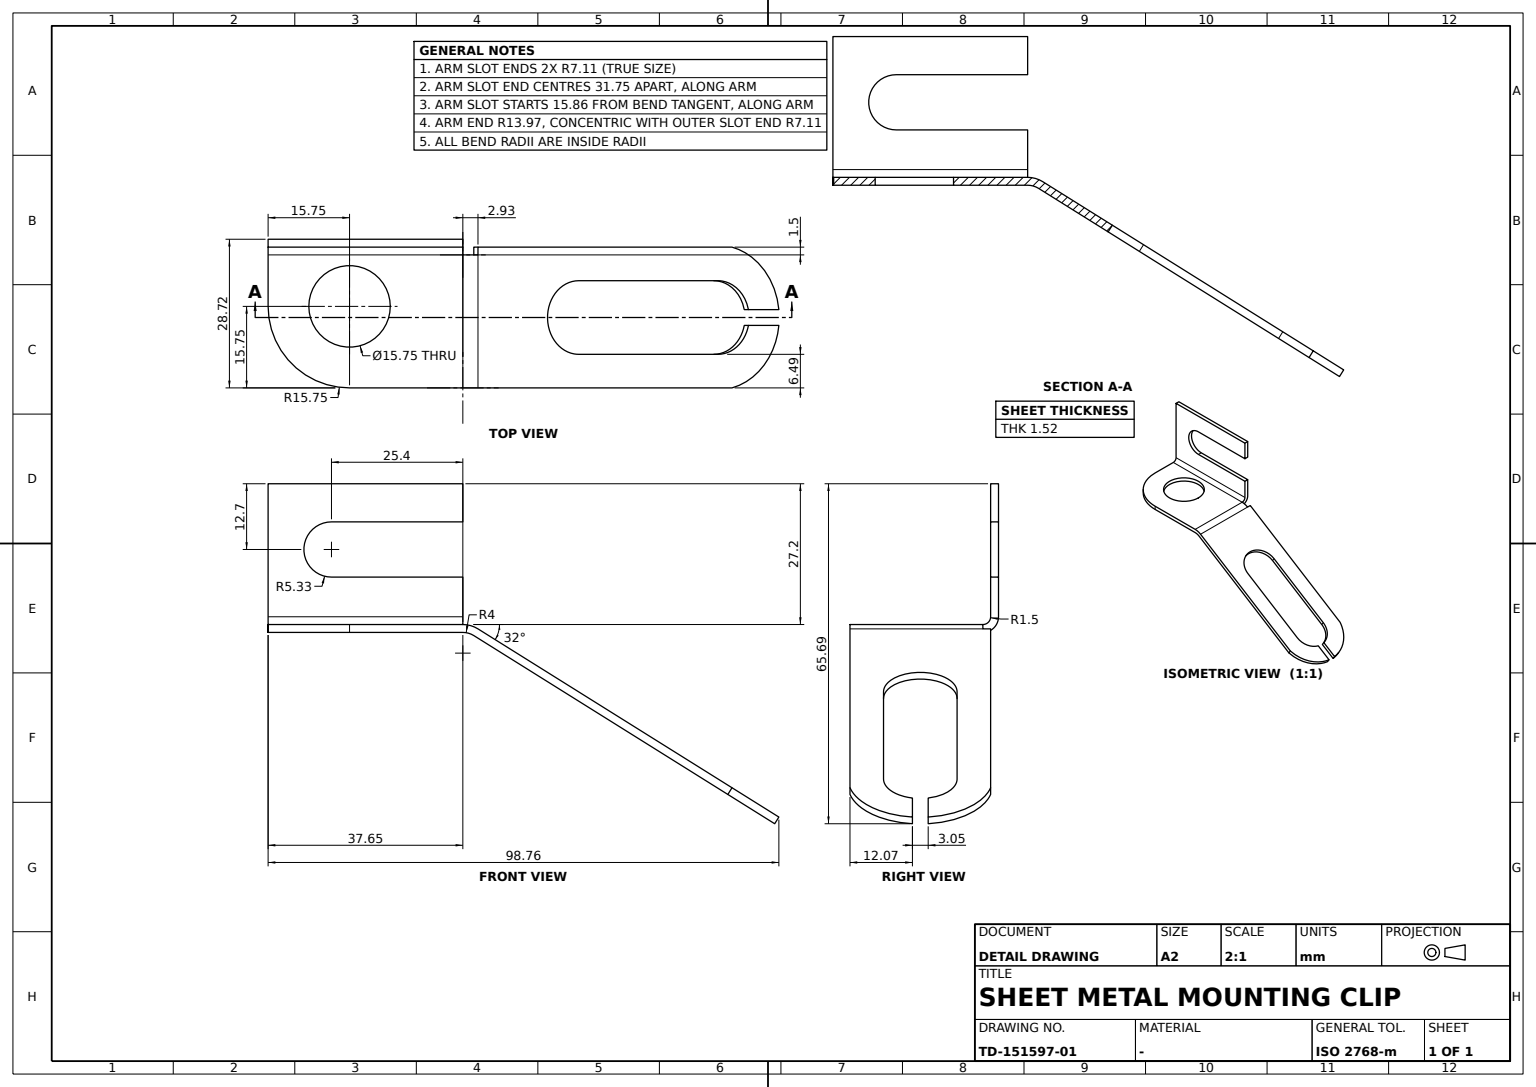
ISO-10303-21;
HEADER;
FILE_DESCRIPTION((''),'2;1');
FILE_NAME('','',(''),(''),'','','');
FILE_SCHEMA(('AUTOMOTIVE_DESIGN'));
ENDSEC;
DATA;
#1=APPLICATION_CONTEXT('');
#2=PRODUCT_CONTEXT('',#1,'mechanical');
#3=PRODUCT('','','',(#2));
#4=PRODUCT_DEFINITION_FORMATION('','',#3);
#5=PRODUCT_DEFINITION_CONTEXT('',#1,'design');
#6=PRODUCT_DEFINITION('','',#4,#5);
#7=PRODUCT_DEFINITION_SHAPE('','',#6);
#8=(LENGTH_UNIT()NAMED_UNIT(*)SI_UNIT(.MILLI.,.METRE.));
#9=(NAMED_UNIT(*)PLANE_ANGLE_UNIT()SI_UNIT($,.RADIAN.));
#10=(NAMED_UNIT(*)SI_UNIT($,.STERADIAN.)SOLID_ANGLE_UNIT());
#11=UNCERTAINTY_MEASURE_WITH_UNIT(LENGTH_MEASURE(0.005),#8,'distance_accuracy_value','');
#12=(GEOMETRIC_REPRESENTATION_CONTEXT(3)GLOBAL_UNCERTAINTY_ASSIGNED_CONTEXT((#11))GLOBAL_UNIT_ASSIGNED_CONTEXT((#8,#9,#10))REPRESENTATION_CONTEXT('',''));
#13=CARTESIAN_POINT('',(-26.546982,13.5977,21.356));
#14=VERTEX_POINT('',#13);
#15=CARTESIAN_POINT('',(-26.546982,15.1217,21.356));
#16=VERTEX_POINT('',#15);
#17=DIRECTION('',(0.,1.,0.));
#18=VECTOR('',#17,1000.);
#19=LINE('',#13,#18);
#20=EDGE_CURVE('',#14,#16,#19,.T.);
#21=ORIENTED_EDGE('',*,*,#20,.F.);
#22=CARTESIAN_POINT('',(-26.546982,13.5977,10.688));
#23=VERTEX_POINT('',#22);
#24=CARTESIAN_POINT('',(-26.546982,13.5977,16.022));
#25=DIRECTION('',(0.,0.,1.));
#26=AXIS2_PLACEMENT_3D('',#24,#17,#25);
#27=CIRCLE('',#26,5.334);
#28=EDGE_CURVE('',#23,#14,#27,.T.);
#29=ORIENTED_EDGE('',*,*,#28,.F.);
#30=CARTESIAN_POINT('',(-26.546982,15.1217,10.688));
#31=VERTEX_POINT('',#30);
#32=LINE('',#22,#18);
#33=EDGE_CURVE('',#31,#23,#32,.F.);
#34=ORIENTED_EDGE('',*,*,#33,.F.);
#35=CARTESIAN_POINT('',(-26.546982,15.1217,16.022));
#36=AXIS2_PLACEMENT_3D('',#35,#17,#25);
#37=CIRCLE('',#36,5.334);
#38=EDGE_CURVE('',#31,#16,#37,.T.);
#39=ORIENTED_EDGE('',*,*,#38,.T.);
#40=EDGE_LOOP('',(#21,#29,#34,#39));
#41=FACE_BOUND('',#40,.T.);
#42=DIRECTION('',(-1.,0.,0.));
#43=AXIS2_PLACEMENT_3D('',#24,#17,#42);
#44=CYLINDRICAL_SURFACE('',#43,5.334);
#45=ADVANCED_FACE('',(#41),#44,.F.);
#46=CARTESIAN_POINT('',(1.780292,-13.5977,0.684618));
#47=VERTEX_POINT('',#46);
#48=CARTESIAN_POINT('',(50.901496,-13.5977,-30.009717));
#49=VERTEX_POINT('',#48);
#50=CARTESIAN_POINT('',(31.407897,-13.5977,-17.828764));
#51=DIRECTION('',(0.848048096,0.,-0.529919264));
#52=VECTOR('',#51,1000.);
#53=LINE('',#50,#52);
#54=EDGE_CURVE('',#47,#49,#53,.T.);
#55=ORIENTED_EDGE('',*,*,#54,.T.);
#56=CARTESIAN_POINT('',(59.961161,-1.524,-35.670824));
#57=VERTEX_POINT('',#56);
#58=CARTESIAN_POINT('',(48.184636,0.,-28.312035));
#59=DIRECTION('',(0.529919264,0.,0.848048096));
#60=AXIS2_PLACEMENT_3D('',#58,#59,#51);
#61=CIRCLE('',#60,13.97);
#62=EDGE_CURVE('',#49,#57,#61,.T.);
#63=ORIENTED_EDGE('',*,*,#62,.T.);
#64=CARTESIAN_POINT('',(54.075853,-1.524,-31.993275));
#65=VERTEX_POINT('',#64);
#66=CARTESIAN_POINT('',(0.807597,-1.524,1.292425));
#67=DIRECTION('',(-0.848048096,0.,0.529919264));
#68=VECTOR('',#67,1000.);
#69=LINE('',#66,#68);
#70=EDGE_CURVE('',#57,#65,#69,.T.);
#71=ORIENTED_EDGE('',*,*,#70,.T.);
#72=CARTESIAN_POINT('',(48.184636,-7.112,-28.312035));
#73=VERTEX_POINT('',#72);
#74=CIRCLE('',#60,7.112);
#75=EDGE_CURVE('',#65,#73,#74,.F.);
#76=ORIENTED_EDGE('',*,*,#75,.T.);
#77=CARTESIAN_POINT('',(21.259109,-7.112,-11.487098));
#78=VERTEX_POINT('',#77);
#79=CARTESIAN_POINT('',(34.721873,-7.112,-19.899566));
#80=LINE('',#79,#68);
#81=EDGE_CURVE('',#73,#78,#80,.T.);
#82=ORIENTED_EDGE('',*,*,#81,.T.);
#83=CARTESIAN_POINT('',(21.259109,7.112,-11.487098));
#84=VERTEX_POINT('',#83);
#85=CARTESIAN_POINT('',(21.259109,0.,-11.487098));
#86=AXIS2_PLACEMENT_3D('',#85,#59,#51);
#87=CIRCLE('',#86,7.112);
#88=EDGE_CURVE('',#78,#84,#87,.F.);
#89=ORIENTED_EDGE('',*,*,#88,.T.);
#90=CARTESIAN_POINT('',(48.184636,7.112,-28.312035));
#91=VERTEX_POINT('',#90);
#92=CARTESIAN_POINT('',(34.721873,7.112,-19.899566));
#93=LINE('',#92,#52);
#94=EDGE_CURVE('',#84,#91,#93,.T.);
#95=ORIENTED_EDGE('',*,*,#94,.T.);
#96=CARTESIAN_POINT('',(54.075853,1.524,-31.993275));
#97=VERTEX_POINT('',#96);
#98=EDGE_CURVE('',#91,#97,#74,.F.);
#99=ORIENTED_EDGE('',*,*,#98,.T.);
#100=CARTESIAN_POINT('',(59.961161,1.524,-35.670824));
#101=VERTEX_POINT('',#100);
#102=CARTESIAN_POINT('',(57.018507,1.524,-33.83205));
#103=LINE('',#102,#52);
#104=EDGE_CURVE('',#97,#101,#103,.T.);
#105=ORIENTED_EDGE('',*,*,#104,.T.);
#106=CARTESIAN_POINT('',(50.901496,13.5977,-30.009717));
#107=VERTEX_POINT('',#106);
#108=EDGE_CURVE('',#107,#101,#61,.F.);
#109=ORIENTED_EDGE('',*,*,#108,.F.);
#110=CARTESIAN_POINT('',(1.780292,13.5977,0.684618));
#111=VERTEX_POINT('',#110);
#112=CARTESIAN_POINT('',(31.407897,13.5977,-17.828764));
#113=LINE('',#112,#52);
#114=EDGE_CURVE('',#111,#107,#113,.T.);
#115=ORIENTED_EDGE('',*,*,#114,.F.);
#116=CARTESIAN_POINT('',(1.780292,12.0977,0.684618));
#117=VERTEX_POINT('',#116);
#118=CARTESIAN_POINT('',(1.780292,0.,0.684618));
#119=DIRECTION('',(0.,-1.,0.));
#120=VECTOR('',#119,1000.);
#121=LINE('',#118,#120);
#122=EDGE_CURVE('',#111,#117,#121,.T.);
#123=ORIENTED_EDGE('',*,*,#122,.T.);
#124=LINE('',#118,#18);
#125=EDGE_CURVE('',#47,#117,#124,.T.);
#126=ORIENTED_EDGE('',*,*,#125,.F.);
#127=EDGE_LOOP('',(#55,#63,#71,#76,#82,#89,#95,#99,#105,#109,#115,#123,#126));
#128=FACE_BOUND('',#127,.T.);
#129=CARTESIAN_POINT('',(0.807597,0.,1.292425));
#130=AXIS2_PLACEMENT_3D('',#129,#59,#51);
#131=PLANE('',#130);
#132=ADVANCED_FACE('',(#128),#131,.T.);
#133=ORIENTED_EDGE('',*,*,#88,.F.);
#134=CARTESIAN_POINT('',(20.451512,-7.112,-12.779523));
#135=VERTEX_POINT('',#134);
#136=VECTOR('',#59,1000.);
#137=LINE('',#77,#136);
#138=EDGE_CURVE('',#135,#78,#137,.T.);
#139=ORIENTED_EDGE('',*,*,#138,.F.);
#140=CARTESIAN_POINT('',(20.451512,7.112,-12.779523));
#141=VERTEX_POINT('',#140);
#142=CARTESIAN_POINT('',(20.451512,0.,-12.779523));
#143=AXIS2_PLACEMENT_3D('',#142,#59,#51);
#144=CIRCLE('',#143,7.112);
#145=EDGE_CURVE('',#135,#141,#144,.F.);
#146=ORIENTED_EDGE('',*,*,#145,.T.);
#147=LINE('',#83,#136);
#148=EDGE_CURVE('',#141,#84,#147,.T.);
#149=ORIENTED_EDGE('',*,*,#148,.T.);
#150=EDGE_LOOP('',(#133,#139,#146,#149));
#151=FACE_BOUND('',#150,.T.);
#152=CYLINDRICAL_SURFACE('',#86,7.112);
#153=ADVANCED_FACE('',(#151),#152,.F.);
#154=ORIENTED_EDGE('',*,*,#38,.F.);
#155=CARTESIAN_POINT('',(-1.146982,15.1217,10.688));
#156=VERTEX_POINT('',#155);
#157=CARTESIAN_POINT('',(0.,15.1217,10.688));
#158=DIRECTION('',(1.,0.,0.));
#159=VECTOR('',#158,1000.);
#160=LINE('',#157,#159);
#161=EDGE_CURVE('',#31,#156,#160,.T.);
#162=ORIENTED_EDGE('',*,*,#161,.T.);
#163=CARTESIAN_POINT('',(-1.146982,15.1217,3.024));
#164=VERTEX_POINT('',#163);
#165=CARTESIAN_POINT('',(-1.146982,15.1217,0.));
#166=DIRECTION('',(0.,0.,-1.));
#167=VECTOR('',#166,1000.);
#168=LINE('',#165,#167);
#169=EDGE_CURVE('',#156,#164,#168,.T.);
#170=ORIENTED_EDGE('',*,*,#169,.T.);
#171=CARTESIAN_POINT('',(-38.8,15.1217,3.024));
#172=VERTEX_POINT('',#171);
#173=CARTESIAN_POINT('',(-19.973491,15.1217,3.024));
#174=LINE('',#173,#159);
#175=EDGE_CURVE('',#172,#164,#174,.T.);
#176=ORIENTED_EDGE('',*,*,#175,.F.);
#177=CARTESIAN_POINT('',(-38.8,15.1217,28.722));
#178=VERTEX_POINT('',#177);
#179=CARTESIAN_POINT('',(-38.8,15.1217,0.));
#180=VECTOR('',#25,1000.);
#181=LINE('',#179,#180);
#182=EDGE_CURVE('',#172,#178,#181,.T.);
#183=ORIENTED_EDGE('',*,*,#182,.T.);
#184=CARTESIAN_POINT('',(-1.146982,15.1217,28.722));
#185=VERTEX_POINT('',#184);
#186=CARTESIAN_POINT('',(0.,15.1217,28.722));
#187=LINE('',#186,#159);
#188=EDGE_CURVE('',#178,#185,#187,.T.);
#189=ORIENTED_EDGE('',*,*,#188,.T.);
#190=CARTESIAN_POINT('',(-1.146982,15.1217,21.356));
#191=VERTEX_POINT('',#190);
#192=EDGE_CURVE('',#185,#191,#168,.T.);
#193=ORIENTED_EDGE('',*,*,#192,.T.);
#194=CARTESIAN_POINT('',(0.,15.1217,21.356));
#195=VECTOR('',#42,1000.);
#196=LINE('',#194,#195);
#197=EDGE_CURVE('',#191,#16,#196,.T.);
#198=ORIENTED_EDGE('',*,*,#197,.T.);
#199=EDGE_LOOP('',(#154,#162,#170,#176,#183,#189,#193,#198));
#200=FACE_BOUND('',#199,.T.);
#201=CARTESIAN_POINT('',(0.,15.1217,0.));
#202=AXIS2_PLACEMENT_3D('',#201,#17,#42);
#203=PLANE('',#202);
#204=ADVANCED_FACE('',(#200),#203,.T.);
#205=ORIENTED_EDGE('',*,*,#108,.T.);
#206=CARTESIAN_POINT('',(59.153564,1.524,-36.963249));
#207=VERTEX_POINT('',#206);
#208=LINE('',#206,#136);
#209=EDGE_CURVE('',#207,#101,#208,.T.);
#210=ORIENTED_EDGE('',*,*,#209,.F.);
#211=CARTESIAN_POINT('',(50.093899,13.5977,-31.302142));
#212=VERTEX_POINT('',#211);
#213=CARTESIAN_POINT('',(47.377039,0.,-29.60446));
#214=AXIS2_PLACEMENT_3D('',#213,#59,#51);
#215=CIRCLE('',#214,13.97);
#216=EDGE_CURVE('',#212,#207,#215,.F.);
#217=ORIENTED_EDGE('',*,*,#216,.F.);
#218=LINE('',#211,#136);
#219=EDGE_CURVE('',#212,#107,#218,.T.);
#220=ORIENTED_EDGE('',*,*,#219,.T.);
#221=EDGE_LOOP('',(#205,#210,#217,#220));
#222=FACE_BOUND('',#221,.T.);
#223=CYLINDRICAL_SURFACE('',#60,13.97);
#224=ADVANCED_FACE('',(#222),#223,.T.);
#225=CARTESIAN_POINT('',(47.377039,-7.112,-29.60446));
#226=VERTEX_POINT('',#225);
#227=CARTESIAN_POINT('',(33.914276,-7.112,-21.191992));
#228=LINE('',#227,#68);
#229=EDGE_CURVE('',#226,#135,#228,.T.);
#230=ORIENTED_EDGE('',*,*,#229,.T.);
#231=ORIENTED_EDGE('',*,*,#138,.T.);
#232=ORIENTED_EDGE('',*,*,#81,.F.);
#233=LINE('',#72,#136);
#234=EDGE_CURVE('',#226,#73,#233,.T.);
#235=ORIENTED_EDGE('',*,*,#234,.F.);
#236=EDGE_LOOP('',(#230,#231,#232,#235));
#237=FACE_BOUND('',#236,.T.);
#238=AXIS2_PLACEMENT_3D('',#79,#119,#158);
#239=PLANE('',#238);
#240=ADVANCED_FACE('',(#237),#239,.F.);
#241=CARTESIAN_POINT('',(-38.8,2.1503,1.524));
#242=VERTEX_POINT('',#241);
#243=CARTESIAN_POINT('',(-23.052,-13.5977,1.524));
#244=VERTEX_POINT('',#243);
#245=CARTESIAN_POINT('',(-23.052,2.1503,1.524));
#246=AXIS2_PLACEMENT_3D('',#245,#25,#158);
#247=CIRCLE('',#246,15.748);
#248=EDGE_CURVE('',#242,#244,#247,.T.);
#249=ORIENTED_EDGE('',*,*,#248,.T.);
#250=CARTESIAN_POINT('',(-1.146982,-13.5977,1.524));
#251=VERTEX_POINT('',#250);
#252=CARTESIAN_POINT('',(0.,-13.5977,1.524));
#253=LINE('',#252,#195);
#254=EDGE_CURVE('',#244,#251,#253,.F.);
#255=ORIENTED_EDGE('',*,*,#254,.T.);
#256=CARTESIAN_POINT('',(-1.146982,12.0977,1.524));
#257=VERTEX_POINT('',#256);
#258=CARTESIAN_POINT('',(-1.146982,0.,1.524));
#259=LINE('',#258,#18);
#260=EDGE_CURVE('',#251,#257,#259,.T.);
#261=ORIENTED_EDGE('',*,*,#260,.T.);
#262=CARTESIAN_POINT('',(-38.8,12.0977,1.524));
#263=VERTEX_POINT('',#262);
#264=CARTESIAN_POINT('',(-19.973491,12.0977,1.524));
#265=LINE('',#264,#159);
#266=EDGE_CURVE('',#263,#257,#265,.T.);
#267=ORIENTED_EDGE('',*,*,#266,.F.);
#268=CARTESIAN_POINT('',(-38.8,0.,1.524));
#269=LINE('',#268,#120);
#270=EDGE_CURVE('',#263,#242,#269,.T.);
#271=ORIENTED_EDGE('',*,*,#270,.T.);
#272=EDGE_LOOP('',(#249,#255,#261,#267,#271));
#273=FACE_BOUND('',#272,.T.);
#274=CARTESIAN_POINT('',(-15.178,2.1503,1.524));
#275=VERTEX_POINT('',#274);
#276=CIRCLE('',#246,7.874);
#277=EDGE_CURVE('',#275,#275,#276,.T.);
#278=ORIENTED_EDGE('',*,*,#277,.F.);
#279=EDGE_LOOP('',(#278));
#280=FACE_BOUND('',#279,.T.);
#281=CARTESIAN_POINT('',(0.,0.,1.524));
#282=AXIS2_PLACEMENT_3D('',#281,#25,#17);
#283=PLANE('',#282);
#284=ADVANCED_FACE('',(#273,#280),#283,.T.);
#285=CARTESIAN_POINT('',(-1.146982,13.5977,3.024));
#286=VERTEX_POINT('',#285);
#287=LINE('',#285,#18);
#288=EDGE_CURVE('',#164,#286,#287,.F.);
#289=ORIENTED_EDGE('',*,*,#288,.F.);
#290=ORIENTED_EDGE('',*,*,#169,.F.);
#291=CARTESIAN_POINT('',(-1.146982,13.5977,10.688));
#292=VERTEX_POINT('',#291);
#293=LINE('',#291,#120);
#294=EDGE_CURVE('',#156,#292,#293,.T.);
#295=ORIENTED_EDGE('',*,*,#294,.T.);
#296=CARTESIAN_POINT('',(-1.146982,13.5977,-18.474977));
#297=LINE('',#296,#167);
#298=EDGE_CURVE('',#292,#286,#297,.T.);
#299=ORIENTED_EDGE('',*,*,#298,.T.);
#300=EDGE_LOOP('',(#289,#290,#295,#299));
#301=FACE_BOUND('',#300,.T.);
#302=AXIS2_PLACEMENT_3D('',#291,#158,#166);
#303=PLANE('',#302);
#304=ADVANCED_FACE('',(#301),#303,.T.);
#305=CARTESIAN_POINT('',(0.972696,13.5977,-0.607808));
#306=VERTEX_POINT('',#305);
#307=CARTESIAN_POINT('',(1.376494,13.5977,0.038405));
#308=LINE('',#307,#136);
#309=EDGE_CURVE('',#306,#111,#308,.T.);
#310=ORIENTED_EDGE('',*,*,#309,.T.);
#311=ORIENTED_EDGE('',*,*,#114,.T.);
#312=ORIENTED_EDGE('',*,*,#219,.F.);
#313=CARTESIAN_POINT('',(30.6003,13.5977,-19.12119));
#314=LINE('',#313,#52);
#315=EDGE_CURVE('',#306,#212,#314,.T.);
#316=ORIENTED_EDGE('',*,*,#315,.F.);
#317=EDGE_LOOP('',(#310,#311,#312,#316));
#318=FACE_BOUND('',#317,.T.);
#319=CARTESIAN_POINT('',(31.004098,13.5977,-18.474977));
#320=AXIS2_PLACEMENT_3D('',#319,#17,#158);
#321=PLANE('',#320);
#322=ADVANCED_FACE('',(#318),#321,.T.);
#323=ORIENTED_EDGE('',*,*,#33,.T.);
#324=CARTESIAN_POINT('',(31.004098,13.5977,10.688));
#325=LINE('',#324,#159);
#326=EDGE_CURVE('',#23,#292,#325,.T.);
#327=ORIENTED_EDGE('',*,*,#326,.T.);
#328=ORIENTED_EDGE('',*,*,#294,.F.);
#329=ORIENTED_EDGE('',*,*,#161,.F.);
#330=EDGE_LOOP('',(#323,#327,#328,#329));
#331=FACE_BOUND('',#330,.T.);
#332=AXIS2_PLACEMENT_3D('',#22,#25,#158);
#333=PLANE('',#332);
#334=ADVANCED_FACE('',(#331),#333,.T.);
#335=CARTESIAN_POINT('',(59.153564,-1.524,-36.963249));
#336=VERTEX_POINT('',#335);
#337=LINE('',#335,#136);
#338=EDGE_CURVE('',#336,#57,#337,.T.);
#339=ORIENTED_EDGE('',*,*,#338,.T.);
#340=ORIENTED_EDGE('',*,*,#62,.F.);
#341=CARTESIAN_POINT('',(50.093899,-13.5977,-31.302142));
#342=VERTEX_POINT('',#341);
#343=LINE('',#341,#136);
#344=EDGE_CURVE('',#342,#49,#343,.T.);
#345=ORIENTED_EDGE('',*,*,#344,.F.);
#346=EDGE_CURVE('',#342,#336,#215,.T.);
#347=ORIENTED_EDGE('',*,*,#346,.T.);
#348=EDGE_LOOP('',(#339,#340,#345,#347));
#349=FACE_BOUND('',#348,.T.);
#350=ADVANCED_FACE('',(#349),#223,.T.);
#351=ORIENTED_EDGE('',*,*,#192,.F.);
#352=CARTESIAN_POINT('',(-1.146982,13.5977,28.722));
#353=VERTEX_POINT('',#352);
#354=LINE('',#352,#120);
#355=EDGE_CURVE('',#185,#353,#354,.T.);
#356=ORIENTED_EDGE('',*,*,#355,.T.);
#357=CARTESIAN_POINT('',(-1.146982,13.5977,21.356));
#358=VERTEX_POINT('',#357);
#359=EDGE_CURVE('',#353,#358,#297,.T.);
#360=ORIENTED_EDGE('',*,*,#359,.T.);
#361=LINE('',#357,#120);
#362=EDGE_CURVE('',#191,#358,#361,.T.);
#363=ORIENTED_EDGE('',*,*,#362,.F.);
#364=EDGE_LOOP('',(#351,#356,#360,#363));
#365=FACE_BOUND('',#364,.T.);
#366=ADVANCED_FACE('',(#365),#303,.T.);
#367=CARTESIAN_POINT('',(0.972696,12.0977,-0.607808));
#368=VERTEX_POINT('',#367);
#369=CARTESIAN_POINT('',(-1.146982,12.0977,0.));
#370=VERTEX_POINT('',#369);
#371=CARTESIAN_POINT('',(-1.146982,12.0977,-4.));
#372=AXIS2_PLACEMENT_3D('',#371,#119,#166);
#373=CIRCLE('',#372,4.);
#374=EDGE_CURVE('',#368,#370,#373,.T.);
#375=ORIENTED_EDGE('',*,*,#374,.T.);
#376=LINE('',#369,#180);
#377=EDGE_CURVE('',#370,#257,#376,.T.);
#378=ORIENTED_EDGE('',*,*,#377,.T.);
#379=CIRCLE('',#372,5.524);
#380=EDGE_CURVE('',#117,#257,#379,.T.);
#381=ORIENTED_EDGE('',*,*,#380,.F.);
#382=LINE('',#367,#136);
#383=EDGE_CURVE('',#368,#117,#382,.T.);
#384=ORIENTED_EDGE('',*,*,#383,.F.);
#385=EDGE_LOOP('',(#375,#378,#381,#384));
#386=FACE_BOUND('',#385,.T.);
#387=DIRECTION('',(-0.913545458,0.,0.406736643));
#388=AXIS2_PLACEMENT_3D('',#367,#119,#387);
#389=PLANE('',#388);
#390=ADVANCED_FACE('',(#386),#389,.F.);
#391=CARTESIAN_POINT('',(-15.178,2.1503,0.));
#392=VERTEX_POINT('',#391);
#393=CARTESIAN_POINT('',(-23.052,2.1503,0.));
#394=AXIS2_PLACEMENT_3D('',#393,#25,#158);
#395=CIRCLE('',#394,7.874);
#396=EDGE_CURVE('',#392,#392,#395,.T.);
#397=ORIENTED_EDGE('',*,*,#396,.T.);
#398=EDGE_LOOP('',(#397));
#399=FACE_BOUND('',#398,.T.);
#400=CARTESIAN_POINT('',(-38.8,12.0977,0.));
#401=VERTEX_POINT('',#400);
#402=CARTESIAN_POINT('',(-19.973491,12.0977,0.));
#403=LINE('',#402,#159);
#404=EDGE_CURVE('',#401,#370,#403,.T.);
#405=ORIENTED_EDGE('',*,*,#404,.T.);
#406=CARTESIAN_POINT('',(-1.146982,-13.5977,0.));
#407=VERTEX_POINT('',#406);
#408=CARTESIAN_POINT('',(-1.146982,0.,0.));
#409=LINE('',#408,#18);
#410=EDGE_CURVE('',#407,#370,#409,.T.);
#411=ORIENTED_EDGE('',*,*,#410,.F.);
#412=CARTESIAN_POINT('',(-23.052,-13.5977,0.));
#413=VERTEX_POINT('',#412);
#414=CARTESIAN_POINT('',(0.,-13.5977,0.));
#415=LINE('',#414,#195);
#416=EDGE_CURVE('',#413,#407,#415,.F.);
#417=ORIENTED_EDGE('',*,*,#416,.F.);
#418=CARTESIAN_POINT('',(-38.8,2.1503,0.));
#419=VERTEX_POINT('',#418);
#420=CIRCLE('',#394,15.748);
#421=EDGE_CURVE('',#419,#413,#420,.T.);
#422=ORIENTED_EDGE('',*,*,#421,.F.);
#423=CARTESIAN_POINT('',(-38.8,0.,0.));
#424=LINE('',#423,#120);
#425=EDGE_CURVE('',#401,#419,#424,.T.);
#426=ORIENTED_EDGE('',*,*,#425,.F.);
#427=EDGE_LOOP('',(#405,#411,#417,#422,#426));
#428=FACE_BOUND('',#427,.T.);
#429=CARTESIAN_POINT('',(0.,0.,0.));
#430=AXIS2_PLACEMENT_3D('',#429,#25,#17);
#431=PLANE('',#430);
#432=ADVANCED_FACE('',(#399,#428),#431,.F.);
#433=ORIENTED_EDGE('',*,*,#362,.T.);
#434=CARTESIAN_POINT('',(31.004098,13.5977,21.356));
#435=LINE('',#434,#195);
#436=EDGE_CURVE('',#358,#14,#435,.T.);
#437=ORIENTED_EDGE('',*,*,#436,.T.);
#438=ORIENTED_EDGE('',*,*,#20,.T.);
#439=ORIENTED_EDGE('',*,*,#197,.F.);
#440=EDGE_LOOP('',(#433,#437,#438,#439));
#441=FACE_BOUND('',#440,.T.);
#442=AXIS2_PLACEMENT_3D('',#357,#166,#42);
#443=PLANE('',#442);
#444=ADVANCED_FACE('',(#441),#443,.T.);
#445=ORIENTED_EDGE('',*,*,#404,.F.);
#446=CARTESIAN_POINT('',(-38.8,12.0977,3.024));
#447=AXIS2_PLACEMENT_3D('',#446,#158,#166);
#448=CIRCLE('',#447,3.024);
#449=EDGE_CURVE('',#401,#172,#448,.T.);
#450=ORIENTED_EDGE('',*,*,#449,.T.);
#451=ORIENTED_EDGE('',*,*,#175,.T.);
#452=CARTESIAN_POINT('',(-1.146982,12.0977,3.024));
#453=AXIS2_PLACEMENT_3D('',#452,#158,#166);
#454=CIRCLE('',#453,3.024);
#455=EDGE_CURVE('',#164,#370,#454,.F.);
#456=ORIENTED_EDGE('',*,*,#455,.T.);
#457=EDGE_LOOP('',(#445,#450,#451,#456));
#458=FACE_BOUND('',#457,.T.);
#459=CARTESIAN_POINT('',(-19.973491,12.0977,3.024));
#460=AXIS2_PLACEMENT_3D('',#459,#158,#17);
#461=CYLINDRICAL_SURFACE('',#460,3.024);
#462=ADVANCED_FACE('',(#458),#461,.T.);
#463=ORIENTED_EDGE('',*,*,#455,.F.);
#464=ORIENTED_EDGE('',*,*,#288,.T.);
#465=CIRCLE('',#453,1.5);
#466=EDGE_CURVE('',#286,#257,#465,.F.);
#467=ORIENTED_EDGE('',*,*,#466,.T.);
#468=ORIENTED_EDGE('',*,*,#377,.F.);
#469=EDGE_LOOP('',(#463,#464,#467,#468));
#470=FACE_BOUND('',#469,.T.);
#471=CARTESIAN_POINT('',(-1.146982,13.5977,2.882628));
#472=CARTESIAN_POINT('',(-1.146982,15.1217,2.738995));
#473=CARTESIAN_POINT('',(-1.146982,13.581045,2.741257));
#474=CARTESIAN_POINT('',(-1.146982,15.088124,2.453989));
#475=CARTESIAN_POINT('',(-1.146982,13.547733,2.602502));
#476=CARTESIAN_POINT('',(-1.146982,15.020966,2.174259));
#477=CARTESIAN_POINT('',(-1.146982,13.449049,2.335453));
#478=CARTESIAN_POINT('',(-1.146982,14.822021,1.635889));
#479=CARTESIAN_POINT('',(-1.146982,13.291007,2.098649));
#480=CARTESIAN_POINT('',(-1.146982,14.503408,1.158493));
#481=CARTESIAN_POINT('',(-1.146982,13.198333,1.990141));
#482=CARTESIAN_POINT('',(-1.146982,14.316575,0.93974));
#483=CARTESIAN_POINT('',(-1.146982,12.989167,1.797));
#484=CARTESIAN_POINT('',(-1.146982,13.894898,0.550369));
#485=CARTESIAN_POINT('',(-1.146982,12.740844,1.657756));
#486=CARTESIAN_POINT('',(-1.146982,13.394279,0.269653));
#487=CARTESIAN_POINT('',(-1.146982,12.609009,1.603148));
#488=CARTESIAN_POINT('',(-1.146982,13.128498,0.159563));
#489=CARTESIAN_POINT('',(-1.146982,12.426308,1.551728));
#490=CARTESIAN_POINT('',(-1.146982,12.760173,0.055899));
#491=CARTESIAN_POINT('',(-1.146982,12.238975,1.529552));
#492=CARTESIAN_POINT('',(-1.146982,12.38251,0.011192));
#493=CARTESIAN_POINT('',(-1.146982,12.191948,1.525851));
#494=CARTESIAN_POINT('',(-1.146982,12.287704,0.003731));
#495=CARTESIAN_POINT('',(-1.146982,12.144824,1.524));
#496=CARTESIAN_POINT('',(-1.146982,12.192702,0.));
#497=B_SPLINE_SURFACE_WITH_KNOTS('',5,1,((#285,#163),(#471,#472),(#473,#474),(#475,#476),(#477,#478),(#479,#480),(#481,#482),(#483,#484),(#485,#486),(#487,#488),(#489,#490),(#491,#492),(#493,#494),(#495,#496),(#256,#369)),.RULED_SURF.,.F.,.F.,.F.,(6,3,3,3,6),(2,2),(0.,0.0045,0.009,0.0135,0.015),(0.,0.0015),.UNSPECIFIED.);
#498=ADVANCED_FACE('',(#470),#497,.T.);
#499=CARTESIAN_POINT('',(47.377039,7.112,-29.60446));
#500=VERTEX_POINT('',#499);
#501=CARTESIAN_POINT('',(33.914276,7.112,-21.191992));
#502=LINE('',#501,#52);
#503=EDGE_CURVE('',#141,#500,#502,.T.);
#504=ORIENTED_EDGE('',*,*,#503,.T.);
#505=LINE('',#90,#136);
#506=EDGE_CURVE('',#500,#91,#505,.T.);
#507=ORIENTED_EDGE('',*,*,#506,.T.);
#508=ORIENTED_EDGE('',*,*,#94,.F.);
#509=ORIENTED_EDGE('',*,*,#148,.F.);
#510=EDGE_LOOP('',(#504,#507,#508,#509));
#511=FACE_BOUND('',#510,.T.);
#512=AXIS2_PLACEMENT_3D('',#92,#17,#158);
#513=PLANE('',#512);
#514=ADVANCED_FACE('',(#511),#513,.F.);
#515=CARTESIAN_POINT('',(-38.8,13.5977,28.722));
#516=VERTEX_POINT('',#515);
#517=CARTESIAN_POINT('',(31.004098,13.5977,28.722));
#518=LINE('',#517,#159);
#519=EDGE_CURVE('',#516,#353,#518,.T.);
#520=ORIENTED_EDGE('',*,*,#519,.T.);
#521=ORIENTED_EDGE('',*,*,#355,.F.);
#522=ORIENTED_EDGE('',*,*,#188,.F.);
#523=LINE('',#515,#120);
#524=EDGE_CURVE('',#178,#516,#523,.T.);
#525=ORIENTED_EDGE('',*,*,#524,.T.);
#526=EDGE_LOOP('',(#520,#521,#522,#525));
#527=FACE_BOUND('',#526,.T.);
#528=AXIS2_PLACEMENT_3D('',#515,#25,#158);
#529=PLANE('',#528);
#530=ADVANCED_FACE('',(#527),#529,.T.);
#531=CARTESIAN_POINT('',(53.268256,-1.524,-33.285701));
#532=VERTEX_POINT('',#531);
#533=LINE('',#531,#136);
#534=EDGE_CURVE('',#532,#65,#533,.T.);
#535=ORIENTED_EDGE('',*,*,#534,.F.);
#536=CIRCLE('',#214,7.112);
#537=EDGE_CURVE('',#532,#226,#536,.F.);
#538=ORIENTED_EDGE('',*,*,#537,.T.);
#539=ORIENTED_EDGE('',*,*,#234,.T.);
#540=ORIENTED_EDGE('',*,*,#75,.F.);
#541=EDGE_LOOP('',(#535,#538,#539,#540));
#542=FACE_BOUND('',#541,.T.);
#543=CYLINDRICAL_SURFACE('',#60,7.112);
#544=ADVANCED_FACE('',(#542),#543,.F.);
#545=ORIENTED_EDGE('',*,*,#277,.T.);
#546=EDGE_LOOP('',(#545));
#547=FACE_BOUND('',#546,.T.);
#548=ORIENTED_EDGE('',*,*,#396,.F.);
#549=EDGE_LOOP('',(#548));
#550=FACE_BOUND('',#549,.T.);
#551=AXIS2_PLACEMENT_3D('',#393,#25,#17);
#552=CYLINDRICAL_SURFACE('',#551,7.874);
#553=ADVANCED_FACE('',(#547,#550),#552,.F.);
#554=ORIENTED_EDGE('',*,*,#309,.F.);
#555=CARTESIAN_POINT('',(0.972696,0.,-0.607808));
#556=LINE('',#555,#120);
#557=EDGE_CURVE('',#306,#368,#556,.T.);
#558=ORIENTED_EDGE('',*,*,#557,.T.);
#559=ORIENTED_EDGE('',*,*,#383,.T.);
#560=ORIENTED_EDGE('',*,*,#122,.F.);
#561=EDGE_LOOP('',(#554,#558,#559,#560));
#562=FACE_BOUND('',#561,.T.);
#563=CARTESIAN_POINT('',(0.972696,12.8477,-0.607808));
#564=AXIS2_PLACEMENT_3D('',#563,#67,#59);
#565=PLANE('',#564);
#566=ADVANCED_FACE('',(#562),#565,.T.);
#567=CARTESIAN_POINT('',(-38.8,13.5977,3.024));
#568=VERTEX_POINT('',#567);
#569=LINE('',#567,#120);
#570=EDGE_CURVE('',#172,#568,#569,.T.);
#571=ORIENTED_EDGE('',*,*,#570,.T.);
#572=CARTESIAN_POINT('',(-38.8,13.5977,-18.474977));
#573=LINE('',#572,#180);
#574=EDGE_CURVE('',#568,#516,#573,.T.);
#575=ORIENTED_EDGE('',*,*,#574,.T.);
#576=ORIENTED_EDGE('',*,*,#524,.F.);
#577=ORIENTED_EDGE('',*,*,#182,.F.);
#578=EDGE_LOOP('',(#571,#575,#576,#577));
#579=FACE_BOUND('',#578,.T.);
#580=CARTESIAN_POINT('',(-38.8,13.5977,0.));
#581=AXIS2_PLACEMENT_3D('',#580,#42,#119);
#582=PLANE('',#581);
#583=ADVANCED_FACE('',(#579),#582,.T.);
#584=ORIENTED_EDGE('',*,*,#380,.T.);
#585=ORIENTED_EDGE('',*,*,#260,.F.);
#586=CARTESIAN_POINT('',(-1.146982,-13.5977,-4.));
#587=AXIS2_PLACEMENT_3D('',#586,#17,#25);
#588=CIRCLE('',#587,5.524);
#589=EDGE_CURVE('',#251,#47,#588,.T.);
#590=ORIENTED_EDGE('',*,*,#589,.T.);
#591=ORIENTED_EDGE('',*,*,#125,.T.);
#592=EDGE_LOOP('',(#584,#585,#590,#591));
#593=FACE_BOUND('',#592,.T.);
#594=CARTESIAN_POINT('',(-1.146982,0.,-4.));
#595=AXIS2_PLACEMENT_3D('',#594,#17,#25);
#596=CYLINDRICAL_SURFACE('',#595,5.524);
#597=ADVANCED_FACE('',(#593),#596,.T.);
#598=CARTESIAN_POINT('',(53.268256,1.524,-33.285701));
#599=VERTEX_POINT('',#598);
#600=CARTESIAN_POINT('',(56.21091,1.524,-35.124475));
#601=LINE('',#600,#52);
#602=EDGE_CURVE('',#599,#207,#601,.T.);
#603=ORIENTED_EDGE('',*,*,#602,.T.);
#604=ORIENTED_EDGE('',*,*,#209,.T.);
#605=ORIENTED_EDGE('',*,*,#104,.F.);
#606=CARTESIAN_POINT('',(53.268256,1.524,-33.2857));
#607=LINE('',#606,#136);
#608=EDGE_CURVE('',#599,#97,#607,.T.);
#609=ORIENTED_EDGE('',*,*,#608,.F.);
#610=EDGE_LOOP('',(#603,#604,#605,#609));
#611=FACE_BOUND('',#610,.T.);
#612=AXIS2_PLACEMENT_3D('',#102,#17,#158);
#613=PLANE('',#612);
#614=ADVANCED_FACE('',(#611),#613,.F.);
#615=ORIENTED_EDGE('',*,*,#466,.F.);
#616=CARTESIAN_POINT('',(-19.973491,13.5977,3.024));
#617=LINE('',#616,#159);
#618=EDGE_CURVE('',#568,#286,#617,.T.);
#619=ORIENTED_EDGE('',*,*,#618,.F.);
#620=CIRCLE('',#447,1.5);
#621=EDGE_CURVE('',#263,#568,#620,.T.);
#622=ORIENTED_EDGE('',*,*,#621,.F.);
#623=ORIENTED_EDGE('',*,*,#266,.T.);
#624=EDGE_LOOP('',(#615,#619,#622,#623));
#625=FACE_BOUND('',#624,.T.);
#626=CYLINDRICAL_SURFACE('',#460,1.5);
#627=ADVANCED_FACE('',(#625),#626,.F.);
#628=ORIENTED_EDGE('',*,*,#570,.F.);
#629=ORIENTED_EDGE('',*,*,#449,.F.);
#630=LINE('',#400,#180);
#631=EDGE_CURVE('',#401,#263,#630,.T.);
#632=ORIENTED_EDGE('',*,*,#631,.T.);
#633=ORIENTED_EDGE('',*,*,#621,.T.);
#634=EDGE_LOOP('',(#628,#629,#632,#633));
#635=FACE_BOUND('',#634,.T.);
#636=CARTESIAN_POINT('',(-38.8,13.5977,2.882628));
#637=CARTESIAN_POINT('',(-38.8,15.1217,2.738995));
#638=CARTESIAN_POINT('',(-38.8,13.581045,2.741257));
#639=CARTESIAN_POINT('',(-38.8,15.088124,2.453989));
#640=CARTESIAN_POINT('',(-38.8,13.547733,2.602502));
#641=CARTESIAN_POINT('',(-38.8,15.020966,2.174259));
#642=CARTESIAN_POINT('',(-38.8,13.449049,2.335453));
#643=CARTESIAN_POINT('',(-38.8,14.822021,1.635889));
#644=CARTESIAN_POINT('',(-38.8,13.291007,2.098649));
#645=CARTESIAN_POINT('',(-38.8,14.503408,1.158493));
#646=CARTESIAN_POINT('',(-38.8,13.198333,1.990141));
#647=CARTESIAN_POINT('',(-38.8,14.316575,0.93974));
#648=CARTESIAN_POINT('',(-38.8,12.989167,1.797));
#649=CARTESIAN_POINT('',(-38.8,13.894898,0.550369));
#650=CARTESIAN_POINT('',(-38.8,12.740844,1.657756));
#651=CARTESIAN_POINT('',(-38.8,13.394279,0.269653));
#652=CARTESIAN_POINT('',(-38.8,12.609009,1.603148));
#653=CARTESIAN_POINT('',(-38.8,13.128498,0.159563));
#654=CARTESIAN_POINT('',(-38.8,12.426308,1.551728));
#655=CARTESIAN_POINT('',(-38.8,12.760173,0.055899));
#656=CARTESIAN_POINT('',(-38.8,12.238975,1.529552));
#657=CARTESIAN_POINT('',(-38.8,12.38251,0.011192));
#658=CARTESIAN_POINT('',(-38.8,12.191948,1.525851));
#659=CARTESIAN_POINT('',(-38.8,12.287704,0.003731));
#660=CARTESIAN_POINT('',(-38.8,12.144824,1.524));
#661=CARTESIAN_POINT('',(-38.8,12.192702,0.));
#662=B_SPLINE_SURFACE_WITH_KNOTS('',5,1,((#567,#171),(#636,#637),(#638,#639),(#640,#641),(#642,#643),(#644,#645),(#646,#647),(#648,#649),(#650,#651),(#652,#653),(#654,#655),(#656,#657),(#658,#659),(#660,#661),(#262,#400)),.RULED_SURF.,.F.,.F.,.F.,(6,3,3,3,6),(2,2),(0.,0.0045,0.009,0.0135,0.015),(0.,0.0015),.UNSPECIFIED.);
#663=ADVANCED_FACE('',(#635),#662,.F.);
#664=LINE('',#418,#180);
#665=EDGE_CURVE('',#419,#242,#664,.T.);
#666=ORIENTED_EDGE('',*,*,#665,.F.);
#667=ORIENTED_EDGE('',*,*,#421,.T.);
#668=LINE('',#412,#180);
#669=EDGE_CURVE('',#413,#244,#668,.T.);
#670=ORIENTED_EDGE('',*,*,#669,.T.);
#671=ORIENTED_EDGE('',*,*,#248,.F.);
#672=EDGE_LOOP('',(#666,#667,#670,#671));
#673=FACE_BOUND('',#672,.T.);
#674=CYLINDRICAL_SURFACE('',#551,15.748);
#675=ADVANCED_FACE('',(#673),#674,.T.);
#676=ORIENTED_EDGE('',*,*,#229,.F.);
#677=ORIENTED_EDGE('',*,*,#537,.F.);
#678=CARTESIAN_POINT('',(0.,-1.524,0.));
#679=LINE('',#678,#68);
#680=EDGE_CURVE('',#336,#532,#679,.T.);
#681=ORIENTED_EDGE('',*,*,#680,.F.);
#682=ORIENTED_EDGE('',*,*,#346,.F.);
#683=CARTESIAN_POINT('',(0.972696,-13.5977,-0.607808));
#684=VERTEX_POINT('',#683);
#685=CARTESIAN_POINT('',(30.6003,-13.5977,-19.12119));
#686=LINE('',#685,#52);
#687=EDGE_CURVE('',#684,#342,#686,.T.);
#688=ORIENTED_EDGE('',*,*,#687,.F.);
#689=LINE('',#555,#18);
#690=EDGE_CURVE('',#684,#368,#689,.T.);
#691=ORIENTED_EDGE('',*,*,#690,.T.);
#692=ORIENTED_EDGE('',*,*,#557,.F.);
#693=ORIENTED_EDGE('',*,*,#315,.T.);
#694=ORIENTED_EDGE('',*,*,#216,.T.);
#695=ORIENTED_EDGE('',*,*,#602,.F.);
#696=EDGE_CURVE('',#500,#599,#536,.F.);
#697=ORIENTED_EDGE('',*,*,#696,.F.);
#698=ORIENTED_EDGE('',*,*,#503,.F.);
#699=ORIENTED_EDGE('',*,*,#145,.F.);
#700=EDGE_LOOP('',(#676,#677,#681,#682,#688,#691,#692,#693,#694,#695,#697,#698,#699));
#701=FACE_BOUND('',#700,.T.);
#702=AXIS2_PLACEMENT_3D('',#429,#59,#51);
#703=PLANE('',#702);
#704=ADVANCED_FACE('',(#701),#703,.F.);
#705=ORIENTED_EDGE('',*,*,#631,.F.);
#706=ORIENTED_EDGE('',*,*,#425,.T.);
#707=ORIENTED_EDGE('',*,*,#665,.T.);
#708=ORIENTED_EDGE('',*,*,#270,.F.);
#709=EDGE_LOOP('',(#705,#706,#707,#708));
#710=FACE_BOUND('',#709,.T.);
#711=ADVANCED_FACE('',(#710),#582,.T.);
#712=ORIENTED_EDGE('',*,*,#70,.F.);
#713=ORIENTED_EDGE('',*,*,#338,.F.);
#714=ORIENTED_EDGE('',*,*,#680,.T.);
#715=ORIENTED_EDGE('',*,*,#534,.T.);
#716=EDGE_LOOP('',(#712,#713,#714,#715));
#717=FACE_BOUND('',#716,.T.);
#718=CARTESIAN_POINT('',(57.018507,-1.524,-33.83205));
#719=AXIS2_PLACEMENT_3D('',#718,#17,#158);
#720=PLANE('',#719);
#721=ADVANCED_FACE('',(#717),#720,.T.);
#722=ORIENTED_EDGE('',*,*,#98,.F.);
#723=ORIENTED_EDGE('',*,*,#506,.F.);
#724=ORIENTED_EDGE('',*,*,#696,.T.);
#725=ORIENTED_EDGE('',*,*,#608,.T.);
#726=EDGE_LOOP('',(#722,#723,#724,#725));
#727=FACE_BOUND('',#726,.T.);
#728=ADVANCED_FACE('',(#727),#543,.F.);
#729=ORIENTED_EDGE('',*,*,#690,.F.);
#730=CIRCLE('',#587,4.);
#731=EDGE_CURVE('',#407,#684,#730,.T.);
#732=ORIENTED_EDGE('',*,*,#731,.F.);
#733=ORIENTED_EDGE('',*,*,#410,.T.);
#734=ORIENTED_EDGE('',*,*,#374,.F.);
#735=EDGE_LOOP('',(#729,#732,#733,#734));
#736=FACE_BOUND('',#735,.T.);
#737=CYLINDRICAL_SURFACE('',#595,4.);
#738=ADVANCED_FACE('',(#736),#737,.F.);
#739=ORIENTED_EDGE('',*,*,#28,.T.);
#740=ORIENTED_EDGE('',*,*,#436,.F.);
#741=ORIENTED_EDGE('',*,*,#359,.F.);
#742=ORIENTED_EDGE('',*,*,#519,.F.);
#743=ORIENTED_EDGE('',*,*,#574,.F.);
#744=ORIENTED_EDGE('',*,*,#618,.T.);
#745=ORIENTED_EDGE('',*,*,#298,.F.);
#746=ORIENTED_EDGE('',*,*,#326,.F.);
#747=EDGE_LOOP('',(#739,#740,#741,#742,#743,#744,#745,#746));
#748=FACE_BOUND('',#747,.T.);
#749=ADVANCED_FACE('',(#748),#321,.F.);
#750=ORIENTED_EDGE('',*,*,#254,.F.);
#751=ORIENTED_EDGE('',*,*,#669,.F.);
#752=ORIENTED_EDGE('',*,*,#416,.T.);
#753=ORIENTED_EDGE('',*,*,#731,.T.);
#754=ORIENTED_EDGE('',*,*,#687,.T.);
#755=ORIENTED_EDGE('',*,*,#344,.T.);
#756=ORIENTED_EDGE('',*,*,#54,.F.);
#757=ORIENTED_EDGE('',*,*,#589,.F.);
#758=EDGE_LOOP('',(#750,#751,#752,#753,#754,#755,#756,#757));
#759=FACE_BOUND('',#758,.T.);
#760=CARTESIAN_POINT('',(31.004098,-13.5977,-18.474977));
#761=AXIS2_PLACEMENT_3D('',#760,#17,#158);
#762=PLANE('',#761);
#763=ADVANCED_FACE('',(#759),#762,.F.);
#764=CLOSED_SHELL('',(#45,#132,#153,#204,#224,#240,#284,#304,#322,#334,#350,#366,#390,#432,#444,#462,#498,#514,#530,#544,#553,#566,#583,#597,#614,#627,#663,#675,#704,#711,#721,#728,#738,#749,#763));
#765=MANIFOLD_SOLID_BREP('',#764);
#766=ADVANCED_BREP_SHAPE_REPRESENTATION('',(#765),#12);
#767=SHAPE_DEFINITION_REPRESENTATION(#7,#766);
ENDSEC;
END-ISO-10303-21;
